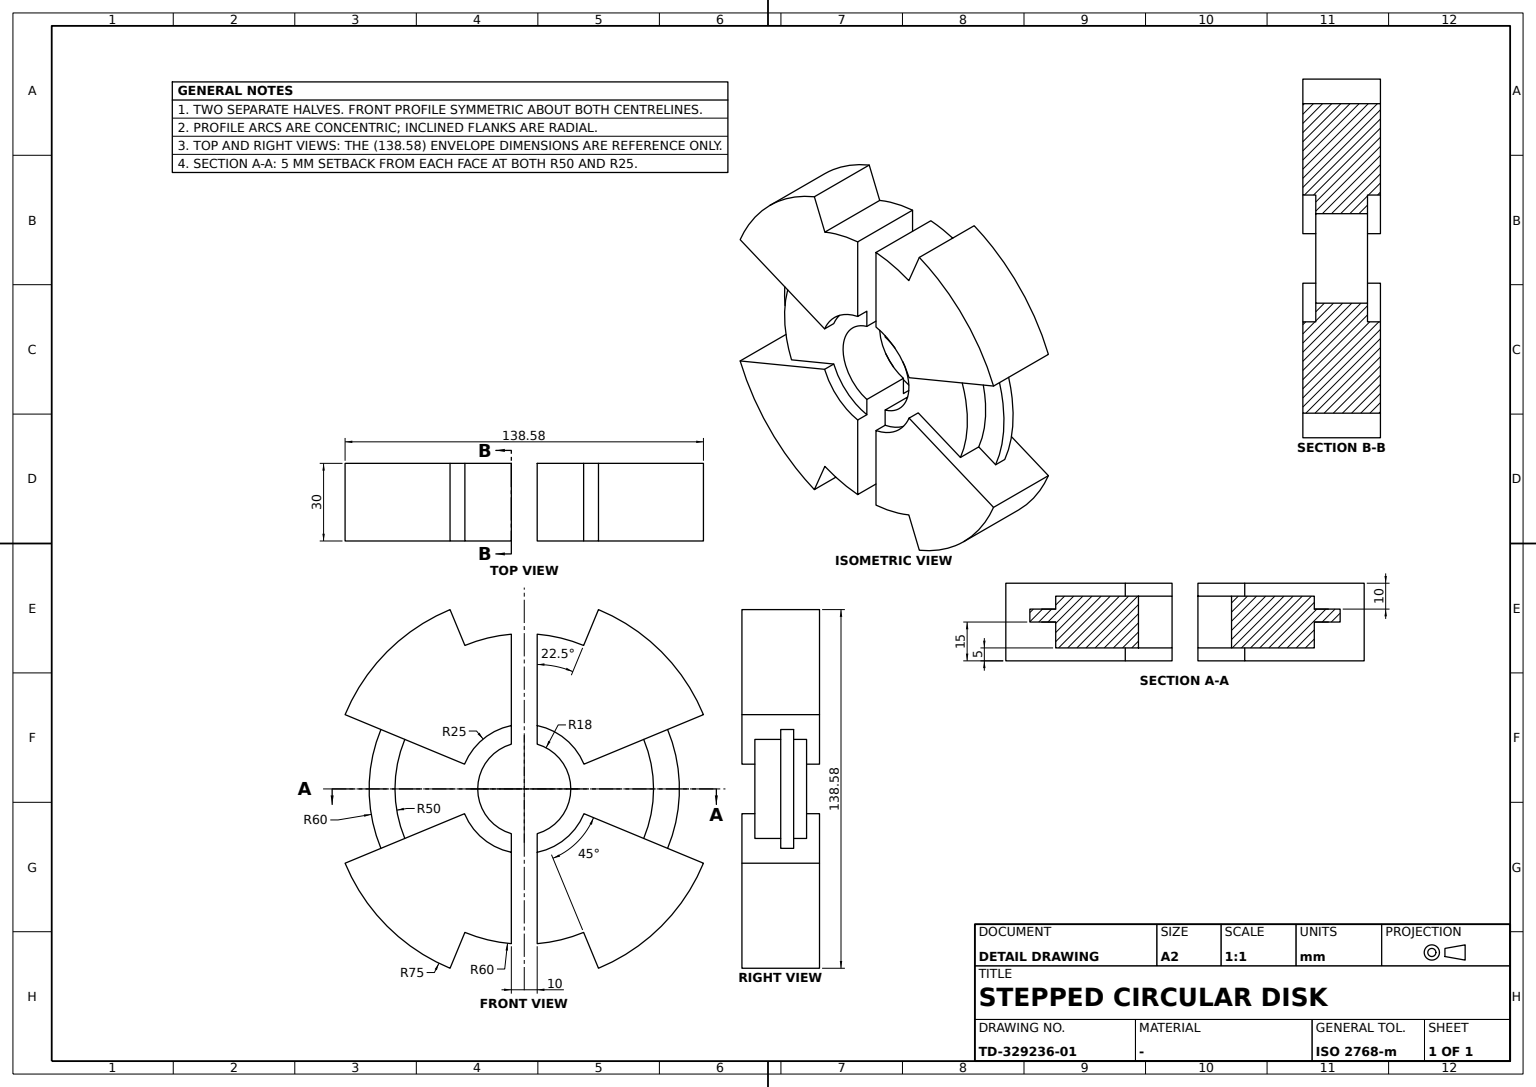
ISO-10303-21;
HEADER;
FILE_DESCRIPTION((''),'2;1');
FILE_NAME('','',(''),(''),'','','');
FILE_SCHEMA(('AUTOMOTIVE_DESIGN'));
ENDSEC;
DATA;
#1=APPLICATION_CONTEXT('');
#2=PRODUCT_CONTEXT('',#1,'mechanical');
#3=PRODUCT('','','',(#2));
#4=PRODUCT_DEFINITION_FORMATION('','',#3);
#5=PRODUCT_DEFINITION_CONTEXT('',#1,'design');
#6=PRODUCT_DEFINITION('','',#4,#5);
#7=PRODUCT_DEFINITION_SHAPE('','',#6);
#8=(LENGTH_UNIT()NAMED_UNIT(*)SI_UNIT(.MILLI.,.METRE.));
#9=(NAMED_UNIT(*)PLANE_ANGLE_UNIT()SI_UNIT($,.RADIAN.));
#10=(NAMED_UNIT(*)SI_UNIT($,.STERADIAN.)SOLID_ANGLE_UNIT());
#11=UNCERTAINTY_MEASURE_WITH_UNIT(LENGTH_MEASURE(0.005),#8,'distance_accuracy_value','');
#12=(GEOMETRIC_REPRESENTATION_CONTEXT(3)GLOBAL_UNCERTAINTY_ASSIGNED_CONTEXT((#11))GLOBAL_UNIT_ASSIGNED_CONTEXT((#8,#9,#10))REPRESENTATION_CONTEXT('',''));
#13=CARTESIAN_POINT('',(-5.,59.791304,-15.));
#14=VERTEX_POINT('',#13);
#15=CARTESIAN_POINT('',(-5.,24.494897,-15.));
#16=VERTEX_POINT('',#15);
#17=CARTESIAN_POINT('',(-5.,0.,-15.));
#18=DIRECTION('',(0.,-1.,0.));
#19=VECTOR('',#18,1000.);
#20=LINE('',#17,#19);
#21=EDGE_CURVE('',#14,#16,#20,.T.);
#22=ORIENTED_EDGE('',*,*,#21,.F.);
#23=CARTESIAN_POINT('',(-5.,59.791304,15.));
#24=VERTEX_POINT('',#23);
#25=CARTESIAN_POINT('',(-5.,59.791304,0.));
#26=DIRECTION('',(0.,0.,1.));
#27=VECTOR('',#26,1000.);
#28=LINE('',#25,#27);
#29=EDGE_CURVE('',#14,#24,#28,.T.);
#30=ORIENTED_EDGE('',*,*,#29,.T.);
#31=CARTESIAN_POINT('',(-5.,24.494897,15.));
#32=VERTEX_POINT('',#31);
#33=CARTESIAN_POINT('',(-5.,0.,15.));
#34=LINE('',#33,#19);
#35=EDGE_CURVE('',#24,#32,#34,.T.);
#36=ORIENTED_EDGE('',*,*,#35,.T.);
#37=CARTESIAN_POINT('',(-5.,24.494897,10.));
#38=VERTEX_POINT('',#37);
#39=LINE('',#37,#27);
#40=EDGE_CURVE('',#38,#32,#39,.T.);
#41=ORIENTED_EDGE('',*,*,#40,.F.);
#42=CARTESIAN_POINT('',(-5.,17.291616,10.));
#43=VERTEX_POINT('',#42);
#44=CARTESIAN_POINT('',(-5.,0.,10.));
#45=LINE('',#44,#19);
#46=EDGE_CURVE('',#38,#43,#45,.T.);
#47=ORIENTED_EDGE('',*,*,#46,.T.);
#48=CARTESIAN_POINT('',(-5.,17.291616,-10.));
#49=VERTEX_POINT('',#48);
#50=LINE('',#48,#27);
#51=EDGE_CURVE('',#43,#49,#50,.F.);
#52=ORIENTED_EDGE('',*,*,#51,.T.);
#53=CARTESIAN_POINT('',(-5.,24.494897,-10.));
#54=VERTEX_POINT('',#53);
#55=CARTESIAN_POINT('',(-5.,0.,-10.));
#56=LINE('',#55,#19);
#57=EDGE_CURVE('',#54,#49,#56,.T.);
#58=ORIENTED_EDGE('',*,*,#57,.F.);
#59=LINE('',#15,#27);
#60=EDGE_CURVE('',#16,#54,#59,.T.);
#61=ORIENTED_EDGE('',*,*,#60,.F.);
#62=EDGE_LOOP('',(#22,#30,#36,#41,#47,#52,#58,#61));
#63=FACE_BOUND('',#62,.T.);
#64=DIRECTION('',(-1.,0.,0.));
#65=AXIS2_PLACEMENT_3D('',#23,#64,#18);
#66=PLANE('',#65);
#67=ADVANCED_FACE('',(#63),#66,.F.);
#68=CARTESIAN_POINT('',(-22.961006,55.432772,-15.));
#69=VERTEX_POINT('',#68);
#70=CARTESIAN_POINT('',(-22.961006,55.432772,15.));
#71=VERTEX_POINT('',#70);
#72=CARTESIAN_POINT('',(-22.961006,55.432772,0.));
#73=LINE('',#72,#27);
#74=EDGE_CURVE('',#69,#71,#73,.T.);
#75=ORIENTED_EDGE('',*,*,#74,.F.);
#76=CARTESIAN_POINT('',(-28.701257,69.290965,-15.));
#77=VERTEX_POINT('',#76);
#78=CARTESIAN_POINT('',(0.,0.,-15.));
#79=DIRECTION('',(0.382683432,-0.923879533,0.));
#80=VECTOR('',#79,1000.);
#81=LINE('',#78,#80);
#82=EDGE_CURVE('',#77,#69,#81,.T.);
#83=ORIENTED_EDGE('',*,*,#82,.F.);
#84=CARTESIAN_POINT('',(-28.701257,69.290965,15.));
#85=VERTEX_POINT('',#84);
#86=CARTESIAN_POINT('',(-28.701257,69.290965,0.));
#87=LINE('',#86,#27);
#88=EDGE_CURVE('',#77,#85,#87,.T.);
#89=ORIENTED_EDGE('',*,*,#88,.T.);
#90=CARTESIAN_POINT('',(0.,0.,15.));
#91=LINE('',#90,#80);
#92=EDGE_CURVE('',#85,#71,#91,.T.);
#93=ORIENTED_EDGE('',*,*,#92,.T.);
#94=EDGE_LOOP('',(#75,#83,#89,#93));
#95=FACE_BOUND('',#94,.T.);
#96=CARTESIAN_POINT('',(22.961006,-55.432772,15.));
#97=DIRECTION('',(-0.923879533,-0.382683432,0.));
#98=AXIS2_PLACEMENT_3D('',#96,#97,#79);
#99=PLANE('',#98);
#100=ADVANCED_FACE('',(#95),#99,.F.);
#101=CARTESIAN_POINT('',(-46.193977,19.134172,10.));
#102=VERTEX_POINT('',#101);
#103=CARTESIAN_POINT('',(-23.096988,9.567086,10.));
#104=VERTEX_POINT('',#103);
#105=DIRECTION('',(0.923879533,-0.382683432,0.));
#106=VECTOR('',#105,1000.);
#107=LINE('',#103,#106);
#108=EDGE_CURVE('',#102,#104,#107,.T.);
#109=ORIENTED_EDGE('',*,*,#108,.F.);
#110=CARTESIAN_POINT('',(-46.193977,-19.134172,10.));
#111=VERTEX_POINT('',#110);
#112=CARTESIAN_POINT('',(0.,0.,10.));
#113=DIRECTION('',(1.,0.,0.));
#114=AXIS2_PLACEMENT_3D('',#112,#26,#113);
#115=CIRCLE('',#114,50.);
#116=EDGE_CURVE('',#102,#111,#115,.T.);
#117=ORIENTED_EDGE('',*,*,#116,.T.);
#118=CARTESIAN_POINT('',(-23.096988,-9.567086,10.));
#119=VERTEX_POINT('',#118);
#120=DIRECTION('',(0.923879533,0.382683432,0.));
#121=VECTOR('',#120,1000.);
#122=LINE('',#112,#121);
#123=EDGE_CURVE('',#111,#119,#122,.T.);
#124=ORIENTED_EDGE('',*,*,#123,.T.);
#125=CARTESIAN_POINT('',(-5.,-24.494897,10.));
#126=VERTEX_POINT('',#125);
#127=CIRCLE('',#114,25.);
#128=EDGE_CURVE('',#119,#126,#127,.T.);
#129=ORIENTED_EDGE('',*,*,#128,.T.);
#130=CARTESIAN_POINT('',(-5.,-17.291616,10.));
#131=VERTEX_POINT('',#130);
#132=EDGE_CURVE('',#131,#126,#45,.T.);
#133=ORIENTED_EDGE('',*,*,#132,.F.);
#134=CIRCLE('',#114,18.);
#135=EDGE_CURVE('',#43,#131,#134,.T.);
#136=ORIENTED_EDGE('',*,*,#135,.F.);
#137=ORIENTED_EDGE('',*,*,#46,.F.);
#138=EDGE_CURVE('',#38,#104,#127,.T.);
#139=ORIENTED_EDGE('',*,*,#138,.T.);
#140=EDGE_LOOP('',(#109,#117,#124,#129,#133,#136,#137,#139));
#141=FACE_BOUND('',#140,.T.);
#142=PLANE('',#114);
#143=ADVANCED_FACE('',(#141),#142,.T.);
#144=CARTESIAN_POINT('',(-23.096988,-9.567086,15.));
#145=VERTEX_POINT('',#144);
#146=CARTESIAN_POINT('',(-5.,-24.494897,15.));
#147=VERTEX_POINT('',#146);
#148=AXIS2_PLACEMENT_3D('',#90,#26,#113);
#149=CIRCLE('',#148,25.);
#150=EDGE_CURVE('',#145,#147,#149,.T.);
#151=ORIENTED_EDGE('',*,*,#150,.T.);
#152=LINE('',#125,#27);
#153=EDGE_CURVE('',#126,#147,#152,.T.);
#154=ORIENTED_EDGE('',*,*,#153,.F.);
#155=ORIENTED_EDGE('',*,*,#128,.F.);
#156=LINE('',#118,#27);
#157=EDGE_CURVE('',#119,#145,#156,.T.);
#158=ORIENTED_EDGE('',*,*,#157,.T.);
#159=EDGE_LOOP('',(#151,#154,#155,#158));
#160=FACE_BOUND('',#159,.T.);
#161=CARTESIAN_POINT('',(0.,0.,0.));
#162=AXIS2_PLACEMENT_3D('',#161,#26,#113);
#163=CYLINDRICAL_SURFACE('',#162,25.);
#164=ADVANCED_FACE('',(#160),#163,.F.);
#165=CARTESIAN_POINT('',(-69.290965,28.701257,-15.));
#166=VERTEX_POINT('',#165);
#167=AXIS2_PLACEMENT_3D('',#78,#26,#113);
#168=CIRCLE('',#167,75.);
#169=EDGE_CURVE('',#77,#166,#168,.T.);
#170=ORIENTED_EDGE('',*,*,#169,.F.);
#171=ORIENTED_EDGE('',*,*,#82,.T.);
#172=CIRCLE('',#167,60.);
#173=EDGE_CURVE('',#14,#69,#172,.T.);
#174=ORIENTED_EDGE('',*,*,#173,.F.);
#175=ORIENTED_EDGE('',*,*,#21,.T.);
#176=CARTESIAN_POINT('',(-23.096988,9.567086,-15.));
#177=VERTEX_POINT('',#176);
#178=CIRCLE('',#167,25.);
#179=EDGE_CURVE('',#16,#177,#178,.T.);
#180=ORIENTED_EDGE('',*,*,#179,.T.);
#181=DIRECTION('',(-0.923879533,0.382683432,0.));
#182=VECTOR('',#181,1000.);
#183=LINE('',#78,#182);
#184=EDGE_CURVE('',#177,#166,#183,.T.);
#185=ORIENTED_EDGE('',*,*,#184,.T.);
#186=EDGE_LOOP('',(#170,#171,#174,#175,#180,#185));
#187=FACE_BOUND('',#186,.T.);
#188=PLANE('',#167);
#189=ADVANCED_FACE('',(#187),#188,.F.);
#190=ORIENTED_EDGE('',*,*,#169,.T.);
#191=CARTESIAN_POINT('',(-69.290965,28.701257,15.));
#192=VERTEX_POINT('',#191);
#193=LINE('',#165,#27);
#194=EDGE_CURVE('',#166,#192,#193,.T.);
#195=ORIENTED_EDGE('',*,*,#194,.T.);
#196=CIRCLE('',#148,75.);
#197=EDGE_CURVE('',#85,#192,#196,.T.);
#198=ORIENTED_EDGE('',*,*,#197,.F.);
#199=ORIENTED_EDGE('',*,*,#88,.F.);
#200=EDGE_LOOP('',(#190,#195,#198,#199));
#201=FACE_BOUND('',#200,.T.);
#202=CYLINDRICAL_SURFACE('',#162,75.);
#203=ADVANCED_FACE('',(#201),#202,.T.);
#204=ORIENTED_EDGE('',*,*,#150,.F.);
#205=CARTESIAN_POINT('',(-69.290965,-28.701257,15.));
#206=VERTEX_POINT('',#205);
#207=CARTESIAN_POINT('',(23.096988,9.567086,15.));
#208=VECTOR('',#97,1000.);
#209=LINE('',#207,#208);
#210=EDGE_CURVE('',#145,#206,#209,.T.);
#211=ORIENTED_EDGE('',*,*,#210,.T.);
#212=CARTESIAN_POINT('',(-28.701257,-69.290965,15.));
#213=VERTEX_POINT('',#212);
#214=EDGE_CURVE('',#206,#213,#196,.T.);
#215=ORIENTED_EDGE('',*,*,#214,.T.);
#216=CARTESIAN_POINT('',(-22.961006,-55.432772,15.));
#217=VERTEX_POINT('',#216);
#218=DIRECTION('',(0.382683432,0.923879533,0.));
#219=VECTOR('',#218,1000.);
#220=LINE('',#90,#219);
#221=EDGE_CURVE('',#213,#217,#220,.T.);
#222=ORIENTED_EDGE('',*,*,#221,.T.);
#223=CARTESIAN_POINT('',(-5.,-59.791304,15.));
#224=VERTEX_POINT('',#223);
#225=CIRCLE('',#148,60.);
#226=EDGE_CURVE('',#217,#224,#225,.T.);
#227=ORIENTED_EDGE('',*,*,#226,.T.);
#228=DIRECTION('',(0.,1.,0.));
#229=VECTOR('',#228,1000.);
#230=LINE('',#23,#229);
#231=EDGE_CURVE('',#147,#224,#230,.F.);
#232=ORIENTED_EDGE('',*,*,#231,.F.);
#233=EDGE_LOOP('',(#204,#211,#215,#222,#227,#232));
#234=FACE_BOUND('',#233,.T.);
#235=PLANE('',#148);
#236=ADVANCED_FACE('',(#234),#235,.T.);
#237=ORIENTED_EDGE('',*,*,#226,.F.);
#238=CARTESIAN_POINT('',(-22.961006,-55.432772,-15.));
#239=VERTEX_POINT('',#238);
#240=CARTESIAN_POINT('',(-22.961006,-55.432772,0.));
#241=LINE('',#240,#27);
#242=EDGE_CURVE('',#217,#239,#241,.F.);
#243=ORIENTED_EDGE('',*,*,#242,.T.);
#244=CARTESIAN_POINT('',(-5.,-59.791304,-15.));
#245=VERTEX_POINT('',#244);
#246=EDGE_CURVE('',#239,#245,#172,.T.);
#247=ORIENTED_EDGE('',*,*,#246,.T.);
#248=CARTESIAN_POINT('',(-5.,-59.791304,0.));
#249=LINE('',#248,#27);
#250=EDGE_CURVE('',#224,#245,#249,.F.);
#251=ORIENTED_EDGE('',*,*,#250,.F.);
#252=EDGE_LOOP('',(#237,#243,#247,#251));
#253=FACE_BOUND('',#252,.T.);
#254=CARTESIAN_POINT('',(0.,0.,-2.5));
#255=AXIS2_PLACEMENT_3D('',#254,#26,#113);
#256=CYLINDRICAL_SURFACE('',#255,60.);
#257=ADVANCED_FACE('',(#253),#256,.T.);
#258=CARTESIAN_POINT('',(-46.193977,-19.134172,0.));
#259=VERTEX_POINT('',#258);
#260=LINE('',#258,#27);
#261=EDGE_CURVE('',#259,#111,#260,.T.);
#262=ORIENTED_EDGE('',*,*,#261,.F.);
#263=CARTESIAN_POINT('',(-55.432772,-22.961006,0.));
#264=VERTEX_POINT('',#263);
#265=LINE('',#161,#121);
#266=EDGE_CURVE('',#264,#259,#265,.T.);
#267=ORIENTED_EDGE('',*,*,#266,.F.);
#268=CARTESIAN_POINT('',(-55.432772,-22.961006,-5.));
#269=VERTEX_POINT('',#268);
#270=LINE('',#268,#27);
#271=EDGE_CURVE('',#269,#264,#270,.T.);
#272=ORIENTED_EDGE('',*,*,#271,.F.);
#273=CARTESIAN_POINT('',(-46.193977,-19.134172,-5.));
#274=VERTEX_POINT('',#273);
#275=CARTESIAN_POINT('',(0.,0.,-5.));
#276=LINE('',#275,#121);
#277=EDGE_CURVE('',#269,#274,#276,.T.);
#278=ORIENTED_EDGE('',*,*,#277,.T.);
#279=CARTESIAN_POINT('',(-46.193977,-19.134172,-10.));
#280=VERTEX_POINT('',#279);
#281=LINE('',#279,#27);
#282=EDGE_CURVE('',#280,#274,#281,.T.);
#283=ORIENTED_EDGE('',*,*,#282,.F.);
#284=CARTESIAN_POINT('',(-23.096988,-9.567086,-10.));
#285=VERTEX_POINT('',#284);
#286=CARTESIAN_POINT('',(0.,0.,-10.));
#287=LINE('',#286,#121);
#288=EDGE_CURVE('',#280,#285,#287,.T.);
#289=ORIENTED_EDGE('',*,*,#288,.T.);
#290=CARTESIAN_POINT('',(-23.096988,-9.567086,-15.));
#291=VERTEX_POINT('',#290);
#292=LINE('',#290,#27);
#293=EDGE_CURVE('',#291,#285,#292,.T.);
#294=ORIENTED_EDGE('',*,*,#293,.F.);
#295=CARTESIAN_POINT('',(-69.290965,-28.701257,-15.));
#296=VERTEX_POINT('',#295);
#297=CARTESIAN_POINT('',(23.096988,9.567086,-15.));
#298=LINE('',#297,#208);
#299=EDGE_CURVE('',#291,#296,#298,.T.);
#300=ORIENTED_EDGE('',*,*,#299,.T.);
#301=LINE('',#295,#27);
#302=EDGE_CURVE('',#296,#206,#301,.T.);
#303=ORIENTED_EDGE('',*,*,#302,.T.);
#304=ORIENTED_EDGE('',*,*,#210,.F.);
#305=ORIENTED_EDGE('',*,*,#157,.F.);
#306=ORIENTED_EDGE('',*,*,#123,.F.);
#307=EDGE_LOOP('',(#262,#267,#272,#278,#283,#289,#294,#300,#303,#304,#305,#306));
#308=FACE_BOUND('',#307,.T.);
#309=CARTESIAN_POINT('',(23.096988,9.567086,0.));
#310=AXIS2_PLACEMENT_3D('',#309,#79,#120);
#311=PLANE('',#310);
#312=ADVANCED_FACE('',(#308),#311,.F.);
#313=ORIENTED_EDGE('',*,*,#271,.T.);
#314=CARTESIAN_POINT('',(-55.432772,22.961006,0.));
#315=VERTEX_POINT('',#314);
#316=CIRCLE('',#162,60.);
#317=EDGE_CURVE('',#315,#264,#316,.T.);
#318=ORIENTED_EDGE('',*,*,#317,.F.);
#319=CARTESIAN_POINT('',(-55.432772,22.961006,-5.));
#320=VERTEX_POINT('',#319);
#321=LINE('',#319,#27);
#322=EDGE_CURVE('',#320,#315,#321,.T.);
#323=ORIENTED_EDGE('',*,*,#322,.F.);
#324=AXIS2_PLACEMENT_3D('',#275,#26,#113);
#325=CIRCLE('',#324,60.);
#326=EDGE_CURVE('',#320,#269,#325,.T.);
#327=ORIENTED_EDGE('',*,*,#326,.T.);
#328=EDGE_LOOP('',(#313,#318,#323,#327));
#329=FACE_BOUND('',#328,.T.);
#330=ADVANCED_FACE('',(#329),#256,.T.);
#331=CARTESIAN_POINT('',(-46.193977,19.134172,-5.));
#332=VERTEX_POINT('',#331);
#333=CIRCLE('',#324,50.);
#334=EDGE_CURVE('',#332,#274,#333,.T.);
#335=ORIENTED_EDGE('',*,*,#334,.F.);
#336=CARTESIAN_POINT('',(-46.193977,19.134172,-10.));
#337=VERTEX_POINT('',#336);
#338=LINE('',#336,#27);
#339=EDGE_CURVE('',#337,#332,#338,.T.);
#340=ORIENTED_EDGE('',*,*,#339,.F.);
#341=AXIS2_PLACEMENT_3D('',#286,#26,#113);
#342=CIRCLE('',#341,50.);
#343=EDGE_CURVE('',#337,#280,#342,.T.);
#344=ORIENTED_EDGE('',*,*,#343,.T.);
#345=ORIENTED_EDGE('',*,*,#282,.T.);
#346=EDGE_LOOP('',(#335,#340,#344,#345));
#347=FACE_BOUND('',#346,.T.);
#348=CYLINDRICAL_SURFACE('',#162,50.);
#349=ADVANCED_FACE('',(#347),#348,.T.);
#350=CARTESIAN_POINT('',(-23.096988,9.567086,-10.));
#351=VERTEX_POINT('',#350);
#352=LINE('',#176,#27);
#353=EDGE_CURVE('',#177,#351,#352,.T.);
#354=ORIENTED_EDGE('',*,*,#353,.F.);
#355=ORIENTED_EDGE('',*,*,#179,.F.);
#356=ORIENTED_EDGE('',*,*,#60,.T.);
#357=CIRCLE('',#341,25.);
#358=EDGE_CURVE('',#54,#351,#357,.T.);
#359=ORIENTED_EDGE('',*,*,#358,.T.);
#360=EDGE_LOOP('',(#354,#355,#356,#359));
#361=FACE_BOUND('',#360,.T.);
#362=ADVANCED_FACE('',(#361),#163,.F.);
#363=ORIENTED_EDGE('',*,*,#250,.T.);
#364=CARTESIAN_POINT('',(-5.,-24.494897,-15.));
#365=VERTEX_POINT('',#364);
#366=LINE('',#13,#229);
#367=EDGE_CURVE('',#365,#245,#366,.F.);
#368=ORIENTED_EDGE('',*,*,#367,.F.);
#369=CARTESIAN_POINT('',(-5.,-24.494897,-10.));
#370=VERTEX_POINT('',#369);
#371=LINE('',#364,#27);
#372=EDGE_CURVE('',#365,#370,#371,.T.);
#373=ORIENTED_EDGE('',*,*,#372,.T.);
#374=CARTESIAN_POINT('',(-5.,-17.291616,-10.));
#375=VERTEX_POINT('',#374);
#376=EDGE_CURVE('',#375,#370,#56,.T.);
#377=ORIENTED_EDGE('',*,*,#376,.F.);
#378=LINE('',#374,#27);
#379=EDGE_CURVE('',#375,#131,#378,.T.);
#380=ORIENTED_EDGE('',*,*,#379,.T.);
#381=ORIENTED_EDGE('',*,*,#132,.T.);
#382=ORIENTED_EDGE('',*,*,#153,.T.);
#383=ORIENTED_EDGE('',*,*,#231,.T.);
#384=EDGE_LOOP('',(#363,#368,#373,#377,#380,#381,#382,#383));
#385=FACE_BOUND('',#384,.T.);
#386=ADVANCED_FACE('',(#385),#66,.F.);
#387=CARTESIAN_POINT('',(-23.096988,9.567086,15.));
#388=VERTEX_POINT('',#387);
#389=LINE('',#103,#27);
#390=EDGE_CURVE('',#104,#388,#389,.T.);
#391=ORIENTED_EDGE('',*,*,#390,.T.);
#392=LINE('',#90,#182);
#393=EDGE_CURVE('',#388,#192,#392,.T.);
#394=ORIENTED_EDGE('',*,*,#393,.T.);
#395=ORIENTED_EDGE('',*,*,#194,.F.);
#396=ORIENTED_EDGE('',*,*,#184,.F.);
#397=ORIENTED_EDGE('',*,*,#353,.T.);
#398=LINE('',#350,#106);
#399=EDGE_CURVE('',#337,#351,#398,.T.);
#400=ORIENTED_EDGE('',*,*,#399,.F.);
#401=ORIENTED_EDGE('',*,*,#339,.T.);
#402=CARTESIAN_POINT('',(-23.096988,9.567086,-5.));
#403=LINE('',#402,#106);
#404=EDGE_CURVE('',#320,#332,#403,.T.);
#405=ORIENTED_EDGE('',*,*,#404,.F.);
#406=ORIENTED_EDGE('',*,*,#322,.T.);
#407=CARTESIAN_POINT('',(-46.193977,19.134172,0.));
#408=VERTEX_POINT('',#407);
#409=CARTESIAN_POINT('',(-23.096988,9.567086,0.));
#410=LINE('',#409,#106);
#411=EDGE_CURVE('',#315,#408,#410,.T.);
#412=ORIENTED_EDGE('',*,*,#411,.T.);
#413=LINE('',#407,#27);
#414=EDGE_CURVE('',#408,#102,#413,.T.);
#415=ORIENTED_EDGE('',*,*,#414,.T.);
#416=ORIENTED_EDGE('',*,*,#108,.T.);
#417=EDGE_LOOP('',(#391,#394,#395,#396,#397,#400,#401,#405,#406,#412,#415,#416));
#418=FACE_BOUND('',#417,.T.);
#419=AXIS2_PLACEMENT_3D('',#409,#218,#181);
#420=PLANE('',#419);
#421=ADVANCED_FACE('',(#418),#420,.F.);
#422=ORIENTED_EDGE('',*,*,#404,.T.);
#423=ORIENTED_EDGE('',*,*,#334,.T.);
#424=ORIENTED_EDGE('',*,*,#277,.F.);
#425=ORIENTED_EDGE('',*,*,#326,.F.);
#426=EDGE_LOOP('',(#422,#423,#424,#425));
#427=FACE_BOUND('',#426,.T.);
#428=PLANE('',#324);
#429=ADVANCED_FACE('',(#427),#428,.F.);
#430=ORIENTED_EDGE('',*,*,#214,.F.);
#431=ORIENTED_EDGE('',*,*,#302,.F.);
#432=CARTESIAN_POINT('',(-28.701257,-69.290965,-15.));
#433=VERTEX_POINT('',#432);
#434=EDGE_CURVE('',#296,#433,#168,.T.);
#435=ORIENTED_EDGE('',*,*,#434,.T.);
#436=CARTESIAN_POINT('',(-28.701257,-69.290965,0.));
#437=LINE('',#436,#27);
#438=EDGE_CURVE('',#433,#213,#437,.T.);
#439=ORIENTED_EDGE('',*,*,#438,.T.);
#440=EDGE_LOOP('',(#430,#431,#435,#439));
#441=FACE_BOUND('',#440,.T.);
#442=ADVANCED_FACE('',(#441),#202,.T.);
#443=ORIENTED_EDGE('',*,*,#135,.T.);
#444=ORIENTED_EDGE('',*,*,#379,.F.);
#445=CIRCLE('',#341,18.);
#446=EDGE_CURVE('',#49,#375,#445,.T.);
#447=ORIENTED_EDGE('',*,*,#446,.F.);
#448=ORIENTED_EDGE('',*,*,#51,.F.);
#449=EDGE_LOOP('',(#443,#444,#447,#448));
#450=FACE_BOUND('',#449,.T.);
#451=CYLINDRICAL_SURFACE('',#162,18.);
#452=ADVANCED_FACE('',(#450),#451,.F.);
#453=ORIENTED_EDGE('',*,*,#358,.F.);
#454=ORIENTED_EDGE('',*,*,#57,.T.);
#455=ORIENTED_EDGE('',*,*,#446,.T.);
#456=ORIENTED_EDGE('',*,*,#376,.T.);
#457=EDGE_CURVE('',#285,#370,#357,.T.);
#458=ORIENTED_EDGE('',*,*,#457,.F.);
#459=ORIENTED_EDGE('',*,*,#288,.F.);
#460=ORIENTED_EDGE('',*,*,#343,.F.);
#461=ORIENTED_EDGE('',*,*,#399,.T.);
#462=EDGE_LOOP('',(#453,#454,#455,#456,#458,#459,#460,#461));
#463=FACE_BOUND('',#462,.T.);
#464=PLANE('',#341);
#465=ADVANCED_FACE('',(#463),#464,.F.);
#466=ORIENTED_EDGE('',*,*,#266,.T.);
#467=CIRCLE('',#162,50.);
#468=EDGE_CURVE('',#408,#259,#467,.T.);
#469=ORIENTED_EDGE('',*,*,#468,.F.);
#470=ORIENTED_EDGE('',*,*,#411,.F.);
#471=ORIENTED_EDGE('',*,*,#317,.T.);
#472=EDGE_LOOP('',(#466,#469,#470,#471));
#473=FACE_BOUND('',#472,.T.);
#474=PLANE('',#162);
#475=ADVANCED_FACE('',(#473),#474,.T.);
#476=ORIENTED_EDGE('',*,*,#372,.F.);
#477=EDGE_CURVE('',#291,#365,#178,.T.);
#478=ORIENTED_EDGE('',*,*,#477,.F.);
#479=ORIENTED_EDGE('',*,*,#293,.T.);
#480=ORIENTED_EDGE('',*,*,#457,.T.);
#481=EDGE_LOOP('',(#476,#478,#479,#480));
#482=FACE_BOUND('',#481,.T.);
#483=ADVANCED_FACE('',(#482),#163,.F.);
#484=EDGE_CURVE('',#24,#71,#225,.T.);
#485=ORIENTED_EDGE('',*,*,#484,.T.);
#486=ORIENTED_EDGE('',*,*,#92,.F.);
#487=ORIENTED_EDGE('',*,*,#197,.T.);
#488=ORIENTED_EDGE('',*,*,#393,.F.);
#489=EDGE_CURVE('',#32,#388,#149,.T.);
#490=ORIENTED_EDGE('',*,*,#489,.F.);
#491=ORIENTED_EDGE('',*,*,#35,.F.);
#492=EDGE_LOOP('',(#485,#486,#487,#488,#490,#491));
#493=FACE_BOUND('',#492,.T.);
#494=ADVANCED_FACE('',(#493),#235,.T.);
#495=ORIENTED_EDGE('',*,*,#173,.T.);
#496=ORIENTED_EDGE('',*,*,#74,.T.);
#497=ORIENTED_EDGE('',*,*,#484,.F.);
#498=ORIENTED_EDGE('',*,*,#29,.F.);
#499=EDGE_LOOP('',(#495,#496,#497,#498));
#500=FACE_BOUND('',#499,.T.);
#501=ADVANCED_FACE('',(#500),#256,.T.);
#502=ORIENTED_EDGE('',*,*,#116,.F.);
#503=ORIENTED_EDGE('',*,*,#414,.F.);
#504=ORIENTED_EDGE('',*,*,#468,.T.);
#505=ORIENTED_EDGE('',*,*,#261,.T.);
#506=EDGE_LOOP('',(#502,#503,#504,#505));
#507=FACE_BOUND('',#506,.T.);
#508=ADVANCED_FACE('',(#507),#348,.T.);
#509=ORIENTED_EDGE('',*,*,#489,.T.);
#510=ORIENTED_EDGE('',*,*,#390,.F.);
#511=ORIENTED_EDGE('',*,*,#138,.F.);
#512=ORIENTED_EDGE('',*,*,#40,.T.);
#513=EDGE_LOOP('',(#509,#510,#511,#512));
#514=FACE_BOUND('',#513,.T.);
#515=ADVANCED_FACE('',(#514),#163,.F.);
#516=ORIENTED_EDGE('',*,*,#221,.F.);
#517=ORIENTED_EDGE('',*,*,#438,.F.);
#518=LINE('',#78,#219);
#519=EDGE_CURVE('',#433,#239,#518,.T.);
#520=ORIENTED_EDGE('',*,*,#519,.T.);
#521=ORIENTED_EDGE('',*,*,#242,.F.);
#522=EDGE_LOOP('',(#516,#517,#520,#521));
#523=FACE_BOUND('',#522,.T.);
#524=CARTESIAN_POINT('',(22.961006,55.432772,15.));
#525=AXIS2_PLACEMENT_3D('',#524,#105,#218);
#526=PLANE('',#525);
#527=ADVANCED_FACE('',(#523),#526,.T.);
#528=ORIENTED_EDGE('',*,*,#519,.F.);
#529=ORIENTED_EDGE('',*,*,#434,.F.);
#530=ORIENTED_EDGE('',*,*,#299,.F.);
#531=ORIENTED_EDGE('',*,*,#477,.T.);
#532=ORIENTED_EDGE('',*,*,#367,.T.);
#533=ORIENTED_EDGE('',*,*,#246,.F.);
#534=EDGE_LOOP('',(#528,#529,#530,#531,#532,#533));
#535=FACE_BOUND('',#534,.T.);
#536=ADVANCED_FACE('',(#535),#188,.F.);
#537=CLOSED_SHELL('',(#67,#100,#143,#164,#189,#203,#236,#257,#312,#330,#349,#362,#386,#421,#429,#442,#452,#465,#475,#483,#494,#501,#508,#515,#527,#536));
#538=MANIFOLD_SOLID_BREP('',#537);
#539=CARTESIAN_POINT('',(5.,-59.791304,-15.));
#540=VERTEX_POINT('',#539);
#541=CARTESIAN_POINT('',(5.,-59.791304,15.));
#542=VERTEX_POINT('',#541);
#543=CARTESIAN_POINT('',(5.,-59.791304,0.));
#544=LINE('',#543,#27);
#545=EDGE_CURVE('',#540,#542,#544,.T.);
#546=ORIENTED_EDGE('',*,*,#545,.F.);
#547=CARTESIAN_POINT('',(22.961006,-55.432772,-15.));
#548=VERTEX_POINT('',#547);
#549=EDGE_CURVE('',#540,#548,#172,.T.);
#550=ORIENTED_EDGE('',*,*,#549,.T.);
#551=VERTEX_POINT('',#96);
#552=CARTESIAN_POINT('',(22.961006,-55.432772,0.));
#553=LINE('',#552,#27);
#554=EDGE_CURVE('',#551,#548,#553,.F.);
#555=ORIENTED_EDGE('',*,*,#554,.F.);
#556=EDGE_CURVE('',#542,#551,#225,.T.);
#557=ORIENTED_EDGE('',*,*,#556,.F.);
#558=EDGE_LOOP('',(#546,#550,#555,#557));
#559=FACE_BOUND('',#558,.T.);
#560=ADVANCED_FACE('',(#559),#256,.T.);
#561=VERTEX_POINT('',#524);
#562=CARTESIAN_POINT('',(22.961006,55.432772,-15.));
#563=VERTEX_POINT('',#562);
#564=CARTESIAN_POINT('',(22.961006,55.432772,0.));
#565=LINE('',#564,#27);
#566=EDGE_CURVE('',#561,#563,#565,.F.);
#567=ORIENTED_EDGE('',*,*,#566,.T.);
#568=CARTESIAN_POINT('',(5.,59.791304,-15.));
#569=VERTEX_POINT('',#568);
#570=EDGE_CURVE('',#563,#569,#172,.T.);
#571=ORIENTED_EDGE('',*,*,#570,.T.);
#572=CARTESIAN_POINT('',(5.,59.791304,15.));
#573=VERTEX_POINT('',#572);
#574=CARTESIAN_POINT('',(5.,59.791304,0.));
#575=LINE('',#574,#27);
#576=EDGE_CURVE('',#573,#569,#575,.F.);
#577=ORIENTED_EDGE('',*,*,#576,.F.);
#578=EDGE_CURVE('',#561,#573,#225,.T.);
#579=ORIENTED_EDGE('',*,*,#578,.F.);
#580=EDGE_LOOP('',(#567,#571,#577,#579));
#581=FACE_BOUND('',#580,.T.);
#582=ADVANCED_FACE('',(#581),#256,.T.);
#583=CARTESIAN_POINT('',(5.,24.494897,10.));
#584=VERTEX_POINT('',#583);
#585=CARTESIAN_POINT('',(5.,24.494897,15.));
#586=VERTEX_POINT('',#585);
#587=LINE('',#583,#27);
#588=EDGE_CURVE('',#584,#586,#587,.T.);
#589=ORIENTED_EDGE('',*,*,#588,.F.);
#590=CARTESIAN_POINT('',(23.096988,9.567086,10.));
#591=VERTEX_POINT('',#590);
#592=EDGE_CURVE('',#591,#584,#127,.T.);
#593=ORIENTED_EDGE('',*,*,#592,.F.);
#594=VERTEX_POINT('',#207);
#595=LINE('',#590,#27);
#596=EDGE_CURVE('',#591,#594,#595,.T.);
#597=ORIENTED_EDGE('',*,*,#596,.T.);
#598=EDGE_CURVE('',#594,#586,#149,.T.);
#599=ORIENTED_EDGE('',*,*,#598,.T.);
#600=EDGE_LOOP('',(#589,#593,#597,#599));
#601=FACE_BOUND('',#600,.T.);
#602=ADVANCED_FACE('',(#601),#163,.F.);
#603=CARTESIAN_POINT('',(46.193977,19.134172,10.));
#604=VERTEX_POINT('',#603);
#605=LINE('',#590,#208);
#606=EDGE_CURVE('',#604,#591,#605,.T.);
#607=ORIENTED_EDGE('',*,*,#606,.T.);
#608=ORIENTED_EDGE('',*,*,#592,.T.);
#609=CARTESIAN_POINT('',(5.,17.291616,10.));
#610=VERTEX_POINT('',#609);
#611=CARTESIAN_POINT('',(5.,0.,10.));
#612=LINE('',#611,#19);
#613=EDGE_CURVE('',#584,#610,#612,.T.);
#614=ORIENTED_EDGE('',*,*,#613,.T.);
#615=CARTESIAN_POINT('',(5.,-17.291616,10.));
#616=VERTEX_POINT('',#615);
#617=EDGE_CURVE('',#616,#610,#134,.T.);
#618=ORIENTED_EDGE('',*,*,#617,.F.);
#619=CARTESIAN_POINT('',(5.,-24.494897,10.));
#620=VERTEX_POINT('',#619);
#621=EDGE_CURVE('',#616,#620,#612,.T.);
#622=ORIENTED_EDGE('',*,*,#621,.T.);
#623=CARTESIAN_POINT('',(23.096988,-9.567086,10.));
#624=VERTEX_POINT('',#623);
#625=EDGE_CURVE('',#620,#624,#127,.T.);
#626=ORIENTED_EDGE('',*,*,#625,.T.);
#627=CARTESIAN_POINT('',(46.193977,-19.134172,10.));
#628=VERTEX_POINT('',#627);
#629=LINE('',#112,#182);
#630=EDGE_CURVE('',#628,#624,#629,.T.);
#631=ORIENTED_EDGE('',*,*,#630,.F.);
#632=EDGE_CURVE('',#628,#604,#115,.T.);
#633=ORIENTED_EDGE('',*,*,#632,.T.);
#634=EDGE_LOOP('',(#607,#608,#614,#618,#622,#626,#631,#633));
#635=FACE_BOUND('',#634,.T.);
#636=ADVANCED_FACE('',(#635),#142,.T.);
#637=CARTESIAN_POINT('',(55.432772,-22.961006,0.));
#638=VERTEX_POINT('',#637);
#639=CARTESIAN_POINT('',(55.432772,22.961006,0.));
#640=VERTEX_POINT('',#639);
#641=EDGE_CURVE('',#638,#640,#316,.T.);
#642=ORIENTED_EDGE('',*,*,#641,.F.);
#643=CARTESIAN_POINT('',(55.432772,-22.961006,-5.));
#644=VERTEX_POINT('',#643);
#645=LINE('',#643,#27);
#646=EDGE_CURVE('',#644,#638,#645,.T.);
#647=ORIENTED_EDGE('',*,*,#646,.F.);
#648=CARTESIAN_POINT('',(55.432772,22.961006,-5.));
#649=VERTEX_POINT('',#648);
#650=EDGE_CURVE('',#644,#649,#325,.T.);
#651=ORIENTED_EDGE('',*,*,#650,.T.);
#652=LINE('',#648,#27);
#653=EDGE_CURVE('',#649,#640,#652,.T.);
#654=ORIENTED_EDGE('',*,*,#653,.T.);
#655=EDGE_LOOP('',(#642,#647,#651,#654));
#656=FACE_BOUND('',#655,.T.);
#657=ADVANCED_FACE('',(#656),#256,.T.);
#658=CARTESIAN_POINT('',(46.193977,-19.134172,-10.));
#659=VERTEX_POINT('',#658);
#660=CARTESIAN_POINT('',(46.193977,19.134172,-10.));
#661=VERTEX_POINT('',#660);
#662=EDGE_CURVE('',#659,#661,#342,.T.);
#663=ORIENTED_EDGE('',*,*,#662,.F.);
#664=CARTESIAN_POINT('',(23.096988,-9.567086,-10.));
#665=VERTEX_POINT('',#664);
#666=LINE('',#286,#182);
#667=EDGE_CURVE('',#659,#665,#666,.T.);
#668=ORIENTED_EDGE('',*,*,#667,.T.);
#669=CARTESIAN_POINT('',(5.,-24.494897,-10.));
#670=VERTEX_POINT('',#669);
#671=EDGE_CURVE('',#670,#665,#357,.T.);
#672=ORIENTED_EDGE('',*,*,#671,.F.);
#673=CARTESIAN_POINT('',(5.,-17.291616,-10.));
#674=VERTEX_POINT('',#673);
#675=CARTESIAN_POINT('',(5.,0.,-10.));
#676=LINE('',#675,#19);
#677=EDGE_CURVE('',#674,#670,#676,.T.);
#678=ORIENTED_EDGE('',*,*,#677,.F.);
#679=CARTESIAN_POINT('',(5.,17.291616,-10.));
#680=VERTEX_POINT('',#679);
#681=EDGE_CURVE('',#674,#680,#445,.T.);
#682=ORIENTED_EDGE('',*,*,#681,.T.);
#683=CARTESIAN_POINT('',(5.,24.494897,-10.));
#684=VERTEX_POINT('',#683);
#685=EDGE_CURVE('',#684,#680,#676,.T.);
#686=ORIENTED_EDGE('',*,*,#685,.F.);
#687=CARTESIAN_POINT('',(23.096988,9.567086,-10.));
#688=VERTEX_POINT('',#687);
#689=EDGE_CURVE('',#688,#684,#357,.T.);
#690=ORIENTED_EDGE('',*,*,#689,.F.);
#691=LINE('',#687,#208);
#692=EDGE_CURVE('',#661,#688,#691,.T.);
#693=ORIENTED_EDGE('',*,*,#692,.F.);
#694=EDGE_LOOP('',(#663,#668,#672,#678,#682,#686,#690,#693));
#695=FACE_BOUND('',#694,.T.);
#696=ADVANCED_FACE('',(#695),#464,.F.);
#697=CARTESIAN_POINT('',(5.,-24.494897,15.));
#698=VERTEX_POINT('',#697);
#699=LINE('',#619,#27);
#700=EDGE_CURVE('',#620,#698,#699,.T.);
#701=ORIENTED_EDGE('',*,*,#700,.T.);
#702=CARTESIAN_POINT('',(23.096988,-9.567086,15.));
#703=VERTEX_POINT('',#702);
#704=EDGE_CURVE('',#698,#703,#149,.T.);
#705=ORIENTED_EDGE('',*,*,#704,.T.);
#706=LINE('',#623,#27);
#707=EDGE_CURVE('',#624,#703,#706,.T.);
#708=ORIENTED_EDGE('',*,*,#707,.F.);
#709=ORIENTED_EDGE('',*,*,#625,.F.);
#710=EDGE_LOOP('',(#701,#705,#708,#709));
#711=FACE_BOUND('',#710,.T.);
#712=ADVANCED_FACE('',(#711),#163,.F.);
#713=CARTESIAN_POINT('',(23.096988,-9.567086,-15.));
#714=VERTEX_POINT('',#713);
#715=LINE('',#713,#27);
#716=EDGE_CURVE('',#714,#665,#715,.T.);
#717=ORIENTED_EDGE('',*,*,#716,.T.);
#718=ORIENTED_EDGE('',*,*,#667,.F.);
#719=CARTESIAN_POINT('',(46.193977,-19.134172,-5.));
#720=VERTEX_POINT('',#719);
#721=LINE('',#658,#27);
#722=EDGE_CURVE('',#659,#720,#721,.T.);
#723=ORIENTED_EDGE('',*,*,#722,.T.);
#724=LINE('',#275,#182);
#725=EDGE_CURVE('',#644,#720,#724,.T.);
#726=ORIENTED_EDGE('',*,*,#725,.F.);
#727=ORIENTED_EDGE('',*,*,#646,.T.);
#728=CARTESIAN_POINT('',(46.193977,-19.134172,0.));
#729=VERTEX_POINT('',#728);
#730=LINE('',#161,#182);
#731=EDGE_CURVE('',#638,#729,#730,.T.);
#732=ORIENTED_EDGE('',*,*,#731,.T.);
#733=LINE('',#728,#27);
#734=EDGE_CURVE('',#729,#628,#733,.T.);
#735=ORIENTED_EDGE('',*,*,#734,.T.);
#736=ORIENTED_EDGE('',*,*,#630,.T.);
#737=ORIENTED_EDGE('',*,*,#707,.T.);
#738=CARTESIAN_POINT('',(69.290965,-28.701257,15.));
#739=VERTEX_POINT('',#738);
#740=LINE('',#387,#106);
#741=EDGE_CURVE('',#703,#739,#740,.T.);
#742=ORIENTED_EDGE('',*,*,#741,.T.);
#743=CARTESIAN_POINT('',(69.290965,-28.701257,-15.));
#744=VERTEX_POINT('',#743);
#745=LINE('',#743,#27);
#746=EDGE_CURVE('',#744,#739,#745,.T.);
#747=ORIENTED_EDGE('',*,*,#746,.F.);
#748=LINE('',#176,#106);
#749=EDGE_CURVE('',#714,#744,#748,.T.);
#750=ORIENTED_EDGE('',*,*,#749,.F.);
#751=EDGE_LOOP('',(#717,#718,#723,#726,#727,#732,#735,#736,#737,#742,#747,#750));
#752=FACE_BOUND('',#751,.T.);
#753=ADVANCED_FACE('',(#752),#420,.T.);
#754=CARTESIAN_POINT('',(28.701257,-69.290965,15.));
#755=VERTEX_POINT('',#754);
#756=EDGE_CURVE('',#551,#755,#91,.T.);
#757=ORIENTED_EDGE('',*,*,#756,.F.);
#758=ORIENTED_EDGE('',*,*,#554,.T.);
#759=CARTESIAN_POINT('',(28.701257,-69.290965,-15.));
#760=VERTEX_POINT('',#759);
#761=EDGE_CURVE('',#548,#760,#81,.T.);
#762=ORIENTED_EDGE('',*,*,#761,.T.);
#763=CARTESIAN_POINT('',(28.701257,-69.290965,0.));
#764=LINE('',#763,#27);
#765=EDGE_CURVE('',#760,#755,#764,.T.);
#766=ORIENTED_EDGE('',*,*,#765,.T.);
#767=EDGE_LOOP('',(#757,#758,#762,#766));
#768=FACE_BOUND('',#767,.T.);
#769=ADVANCED_FACE('',(#768),#99,.T.);
#770=LINE('',#572,#229);
#771=EDGE_CURVE('',#698,#542,#770,.F.);
#772=ORIENTED_EDGE('',*,*,#771,.T.);
#773=ORIENTED_EDGE('',*,*,#556,.T.);
#774=ORIENTED_EDGE('',*,*,#756,.T.);
#775=EDGE_CURVE('',#755,#739,#196,.T.);
#776=ORIENTED_EDGE('',*,*,#775,.T.);
#777=ORIENTED_EDGE('',*,*,#741,.F.);
#778=ORIENTED_EDGE('',*,*,#704,.F.);
#779=EDGE_LOOP('',(#772,#773,#774,#776,#777,#778));
#780=FACE_BOUND('',#779,.T.);
#781=ADVANCED_FACE('',(#780),#235,.T.);
#782=CARTESIAN_POINT('',(69.290965,28.701257,15.));
#783=VERTEX_POINT('',#782);
#784=CARTESIAN_POINT('',(28.701257,69.290965,15.));
#785=VERTEX_POINT('',#784);
#786=EDGE_CURVE('',#783,#785,#196,.T.);
#787=ORIENTED_EDGE('',*,*,#786,.T.);
#788=EDGE_CURVE('',#561,#785,#220,.T.);
#789=ORIENTED_EDGE('',*,*,#788,.F.);
#790=ORIENTED_EDGE('',*,*,#578,.T.);
#791=CARTESIAN_POINT('',(5.,0.,15.));
#792=LINE('',#791,#19);
#793=EDGE_CURVE('',#573,#586,#792,.T.);
#794=ORIENTED_EDGE('',*,*,#793,.T.);
#795=ORIENTED_EDGE('',*,*,#598,.F.);
#796=LINE('',#90,#121);
#797=EDGE_CURVE('',#594,#783,#796,.T.);
#798=ORIENTED_EDGE('',*,*,#797,.T.);
#799=EDGE_LOOP('',(#787,#789,#790,#794,#795,#798));
#800=FACE_BOUND('',#799,.T.);
#801=ADVANCED_FACE('',(#800),#235,.T.);
#802=CARTESIAN_POINT('',(5.,24.494897,-15.));
#803=VERTEX_POINT('',#802);
#804=CARTESIAN_POINT('',(5.,0.,-15.));
#805=LINE('',#804,#19);
#806=EDGE_CURVE('',#569,#803,#805,.T.);
#807=ORIENTED_EDGE('',*,*,#806,.F.);
#808=ORIENTED_EDGE('',*,*,#570,.F.);
#809=CARTESIAN_POINT('',(28.701257,69.290965,-15.));
#810=VERTEX_POINT('',#809);
#811=EDGE_CURVE('',#563,#810,#518,.T.);
#812=ORIENTED_EDGE('',*,*,#811,.T.);
#813=CARTESIAN_POINT('',(69.290965,28.701257,-15.));
#814=VERTEX_POINT('',#813);
#815=EDGE_CURVE('',#814,#810,#168,.T.);
#816=ORIENTED_EDGE('',*,*,#815,.F.);
#817=VERTEX_POINT('',#297);
#818=LINE('',#78,#121);
#819=EDGE_CURVE('',#817,#814,#818,.T.);
#820=ORIENTED_EDGE('',*,*,#819,.F.);
#821=EDGE_CURVE('',#817,#803,#178,.T.);
#822=ORIENTED_EDGE('',*,*,#821,.T.);
#823=EDGE_LOOP('',(#807,#808,#812,#816,#820,#822));
#824=FACE_BOUND('',#823,.T.);
#825=ADVANCED_FACE('',(#824),#188,.F.);
#826=ORIENTED_EDGE('',*,*,#811,.F.);
#827=ORIENTED_EDGE('',*,*,#566,.F.);
#828=ORIENTED_EDGE('',*,*,#788,.T.);
#829=CARTESIAN_POINT('',(28.701257,69.290965,0.));
#830=LINE('',#829,#27);
#831=EDGE_CURVE('',#810,#785,#830,.T.);
#832=ORIENTED_EDGE('',*,*,#831,.F.);
#833=EDGE_LOOP('',(#826,#827,#828,#832));
#834=FACE_BOUND('',#833,.T.);
#835=ADVANCED_FACE('',(#834),#526,.F.);
#836=ORIENTED_EDGE('',*,*,#653,.F.);
#837=CARTESIAN_POINT('',(46.193977,19.134172,-5.));
#838=VERTEX_POINT('',#837);
#839=CARTESIAN_POINT('',(23.096988,9.567086,-5.));
#840=LINE('',#839,#208);
#841=EDGE_CURVE('',#649,#838,#840,.T.);
#842=ORIENTED_EDGE('',*,*,#841,.T.);
#843=LINE('',#660,#27);
#844=EDGE_CURVE('',#661,#838,#843,.T.);
#845=ORIENTED_EDGE('',*,*,#844,.F.);
#846=ORIENTED_EDGE('',*,*,#692,.T.);
#847=LINE('',#297,#27);
#848=EDGE_CURVE('',#817,#688,#847,.T.);
#849=ORIENTED_EDGE('',*,*,#848,.F.);
#850=ORIENTED_EDGE('',*,*,#819,.T.);
#851=LINE('',#813,#27);
#852=EDGE_CURVE('',#814,#783,#851,.T.);
#853=ORIENTED_EDGE('',*,*,#852,.T.);
#854=ORIENTED_EDGE('',*,*,#797,.F.);
#855=ORIENTED_EDGE('',*,*,#596,.F.);
#856=ORIENTED_EDGE('',*,*,#606,.F.);
#857=CARTESIAN_POINT('',(46.193977,19.134172,0.));
#858=VERTEX_POINT('',#857);
#859=LINE('',#857,#27);
#860=EDGE_CURVE('',#858,#604,#859,.T.);
#861=ORIENTED_EDGE('',*,*,#860,.F.);
#862=LINE('',#309,#208);
#863=EDGE_CURVE('',#640,#858,#862,.T.);
#864=ORIENTED_EDGE('',*,*,#863,.F.);
#865=EDGE_LOOP('',(#836,#842,#845,#846,#849,#850,#853,#854,#855,#856,#861,#864));
#866=FACE_BOUND('',#865,.T.);
#867=ADVANCED_FACE('',(#866),#311,.T.);
#868=EDGE_CURVE('',#729,#858,#467,.T.);
#869=ORIENTED_EDGE('',*,*,#868,.F.);
#870=ORIENTED_EDGE('',*,*,#731,.F.);
#871=ORIENTED_EDGE('',*,*,#641,.T.);
#872=ORIENTED_EDGE('',*,*,#863,.T.);
#873=EDGE_LOOP('',(#869,#870,#871,#872));
#874=FACE_BOUND('',#873,.T.);
#875=ADVANCED_FACE('',(#874),#474,.T.);
#876=ORIENTED_EDGE('',*,*,#677,.T.);
#877=CARTESIAN_POINT('',(5.,-24.494897,-15.));
#878=VERTEX_POINT('',#877);
#879=LINE('',#877,#27);
#880=EDGE_CURVE('',#878,#670,#879,.T.);
#881=ORIENTED_EDGE('',*,*,#880,.F.);
#882=LINE('',#568,#229);
#883=EDGE_CURVE('',#878,#540,#882,.F.);
#884=ORIENTED_EDGE('',*,*,#883,.T.);
#885=ORIENTED_EDGE('',*,*,#545,.T.);
#886=ORIENTED_EDGE('',*,*,#771,.F.);
#887=ORIENTED_EDGE('',*,*,#700,.F.);
#888=ORIENTED_EDGE('',*,*,#621,.F.);
#889=LINE('',#673,#27);
#890=EDGE_CURVE('',#616,#674,#889,.F.);
#891=ORIENTED_EDGE('',*,*,#890,.T.);
#892=EDGE_LOOP('',(#876,#881,#884,#885,#886,#887,#888,#891));
#893=FACE_BOUND('',#892,.T.);
#894=AXIS2_PLACEMENT_3D('',#572,#64,#18);
#895=PLANE('',#894);
#896=ADVANCED_FACE('',(#893),#895,.T.);
#897=ORIENTED_EDGE('',*,*,#786,.F.);
#898=ORIENTED_EDGE('',*,*,#852,.F.);
#899=ORIENTED_EDGE('',*,*,#815,.T.);
#900=ORIENTED_EDGE('',*,*,#831,.T.);
#901=EDGE_LOOP('',(#897,#898,#899,#900));
#902=FACE_BOUND('',#901,.T.);
#903=ADVANCED_FACE('',(#902),#202,.T.);
#904=ORIENTED_EDGE('',*,*,#841,.F.);
#905=ORIENTED_EDGE('',*,*,#650,.F.);
#906=ORIENTED_EDGE('',*,*,#725,.T.);
#907=EDGE_CURVE('',#720,#838,#333,.T.);
#908=ORIENTED_EDGE('',*,*,#907,.T.);
#909=EDGE_LOOP('',(#904,#905,#906,#908));
#910=FACE_BOUND('',#909,.T.);
#911=ADVANCED_FACE('',(#910),#428,.F.);
#912=ORIENTED_EDGE('',*,*,#793,.F.);
#913=ORIENTED_EDGE('',*,*,#576,.T.);
#914=ORIENTED_EDGE('',*,*,#806,.T.);
#915=LINE('',#802,#27);
#916=EDGE_CURVE('',#803,#684,#915,.T.);
#917=ORIENTED_EDGE('',*,*,#916,.T.);
#918=ORIENTED_EDGE('',*,*,#685,.T.);
#919=LINE('',#679,#27);
#920=EDGE_CURVE('',#680,#610,#919,.T.);
#921=ORIENTED_EDGE('',*,*,#920,.T.);
#922=ORIENTED_EDGE('',*,*,#613,.F.);
#923=ORIENTED_EDGE('',*,*,#588,.T.);
#924=EDGE_LOOP('',(#912,#913,#914,#917,#918,#921,#922,#923));
#925=FACE_BOUND('',#924,.T.);
#926=ADVANCED_FACE('',(#925),#895,.T.);
#927=ORIENTED_EDGE('',*,*,#860,.T.);
#928=ORIENTED_EDGE('',*,*,#632,.F.);
#929=ORIENTED_EDGE('',*,*,#734,.F.);
#930=ORIENTED_EDGE('',*,*,#868,.T.);
#931=EDGE_LOOP('',(#927,#928,#929,#930));
#932=FACE_BOUND('',#931,.T.);
#933=ADVANCED_FACE('',(#932),#348,.T.);
#934=ORIENTED_EDGE('',*,*,#880,.T.);
#935=ORIENTED_EDGE('',*,*,#671,.T.);
#936=ORIENTED_EDGE('',*,*,#716,.F.);
#937=EDGE_CURVE('',#878,#714,#178,.T.);
#938=ORIENTED_EDGE('',*,*,#937,.F.);
#939=EDGE_LOOP('',(#934,#935,#936,#938));
#940=FACE_BOUND('',#939,.T.);
#941=ADVANCED_FACE('',(#940),#163,.F.);
#942=ORIENTED_EDGE('',*,*,#765,.F.);
#943=EDGE_CURVE('',#760,#744,#168,.T.);
#944=ORIENTED_EDGE('',*,*,#943,.T.);
#945=ORIENTED_EDGE('',*,*,#746,.T.);
#946=ORIENTED_EDGE('',*,*,#775,.F.);
#947=EDGE_LOOP('',(#942,#944,#945,#946));
#948=FACE_BOUND('',#947,.T.);
#949=ADVANCED_FACE('',(#948),#202,.T.);
#950=ORIENTED_EDGE('',*,*,#821,.F.);
#951=ORIENTED_EDGE('',*,*,#848,.T.);
#952=ORIENTED_EDGE('',*,*,#689,.T.);
#953=ORIENTED_EDGE('',*,*,#916,.F.);
#954=EDGE_LOOP('',(#950,#951,#952,#953));
#955=FACE_BOUND('',#954,.T.);
#956=ADVANCED_FACE('',(#955),#163,.F.);
#957=ORIENTED_EDGE('',*,*,#890,.F.);
#958=ORIENTED_EDGE('',*,*,#617,.T.);
#959=ORIENTED_EDGE('',*,*,#920,.F.);
#960=ORIENTED_EDGE('',*,*,#681,.F.);
#961=EDGE_LOOP('',(#957,#958,#959,#960));
#962=FACE_BOUND('',#961,.T.);
#963=ADVANCED_FACE('',(#962),#451,.F.);
#964=ORIENTED_EDGE('',*,*,#844,.T.);
#965=ORIENTED_EDGE('',*,*,#907,.F.);
#966=ORIENTED_EDGE('',*,*,#722,.F.);
#967=ORIENTED_EDGE('',*,*,#662,.T.);
#968=EDGE_LOOP('',(#964,#965,#966,#967));
#969=FACE_BOUND('',#968,.T.);
#970=ADVANCED_FACE('',(#969),#348,.T.);
#971=ORIENTED_EDGE('',*,*,#943,.F.);
#972=ORIENTED_EDGE('',*,*,#761,.F.);
#973=ORIENTED_EDGE('',*,*,#549,.F.);
#974=ORIENTED_EDGE('',*,*,#883,.F.);
#975=ORIENTED_EDGE('',*,*,#937,.T.);
#976=ORIENTED_EDGE('',*,*,#749,.T.);
#977=EDGE_LOOP('',(#971,#972,#973,#974,#975,#976));
#978=FACE_BOUND('',#977,.T.);
#979=ADVANCED_FACE('',(#978),#188,.F.);
#980=CLOSED_SHELL('',(#560,#582,#602,#636,#657,#696,#712,#753,#769,#781,#801,#825,#835,#867,#875,#896,#903,#911,#926,#933,#941,#949,#956,#963,#970,#979));
#981=MANIFOLD_SOLID_BREP('',#980);
#982=ADVANCED_BREP_SHAPE_REPRESENTATION('',(#538,#981),#12);
#983=SHAPE_DEFINITION_REPRESENTATION(#7,#982);
ENDSEC;
END-ISO-10303-21;
